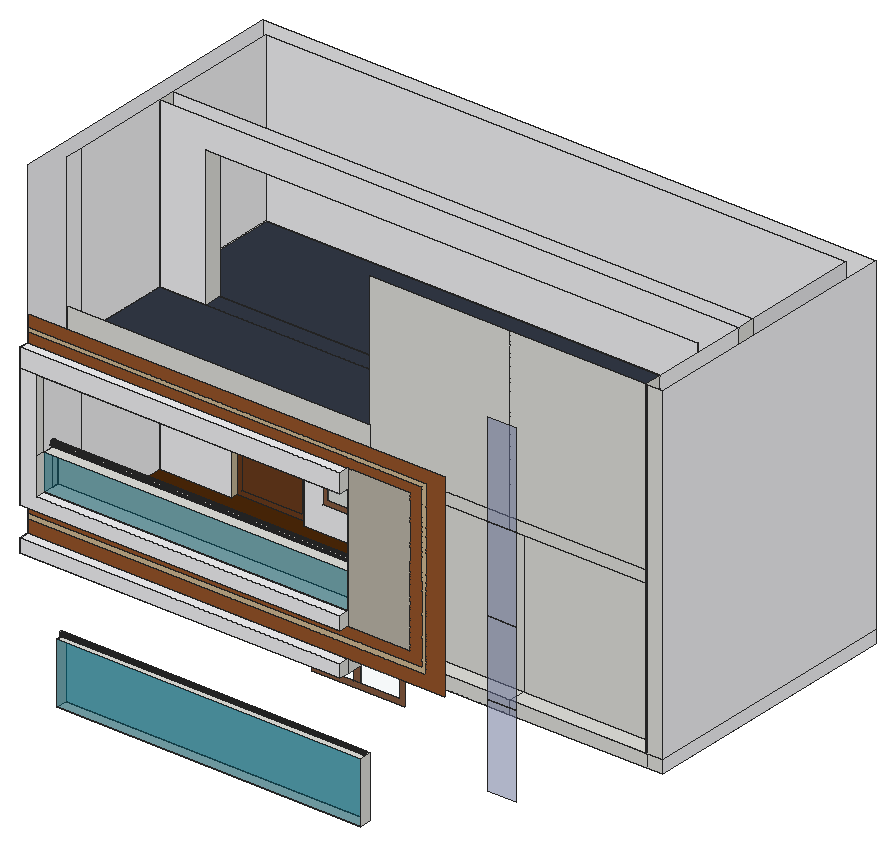
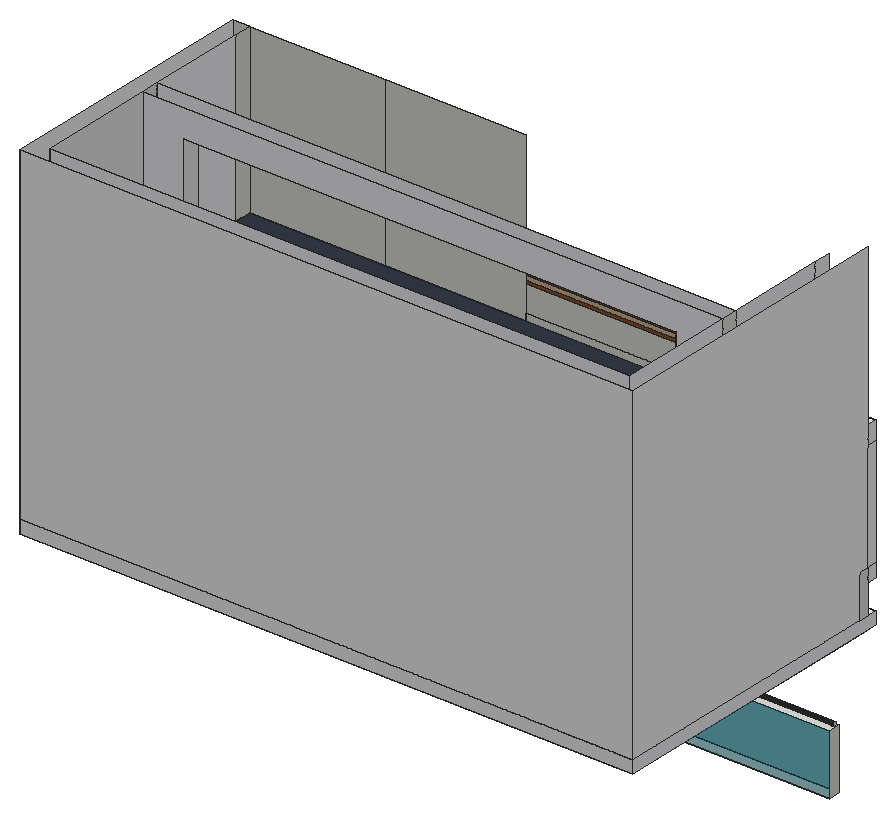
# SketchUp Ruby script. Lengths in inches.
U = 1.inch
M = Sketchup.active_model
def pt(a) = Geom::Point3d.new(a.map { |v| v * U })
def face(e, loops, mat)
  f = e.add_face(loops[0].map { |a| pt(a) })
  loops[1..].each { |l| e.add_face(l.map { |a| pt(a) }).erase! }
  f.material = f.back_material = mat if mat
  f
end
# faces: each face lists its corners as indices into pts; further lists are holes
def faces(e, pts, list, mat = nil) = list.each { |f| face(e, (f[0].is_a?(Array) ? f : [f]).map { |l| l.map { |i| pts[i] } }, mat) }
# xy, xz, yz: faces in a plane at the given z, y or x. An outline is a flat list of corners, or four numbers for a rectangle; further outlines are holes
def ring(l) = l.size == 4 ? [[l[0], l[1]], [l[2], l[1]], [l[2], l[3]], [l[0], l[3]]] : l.each_slice(2).to_a
def flat(e, list, mat, &to3) = list.each { |f| face(e, (f[0].is_a?(Array) ? f : [f]).map { |l| ring(l).map { |u, v| to3.(u, v) } }, mat) }
def xy(e, z, list, mat = nil) = flat(e, list, mat) { |x, y| [x, y, z] }
def xz(e, y, list, mat = nil) = flat(e, list, mat) { |x, z| [x, y, z] }
def yz(e, x, list, mat = nil) = flat(e, list, mat) { |y, z| [x, y, z] }
def lines(e, pts, list) = list.each { |a, b| e.add_line(pt(pts[a]), pt(pts[b])) }
# prism: a flat outline (further loops are holes) pulled along v
def prism(e, loops, v, mat = nil)
  f = face(e, loops, mat); d = Geom::Vector3d.new(v.map { |x| x * U })
  f.pushpull(f.normal.samedirection?(d) ? d.length : -d.length)
end
def box(e, o, s, mat = nil) = prism(e, [[o, [o[0] + s[0], o[1], o[2]], [o[0] + s[0], o[1] + s[1], o[2]], [o[0], o[1] + s[1], o[2]]]], [0, 0, s[2]], mat)
def at(x, y, z, deg = 0) = Geom::Transformation.translation(pt([x, y, z])) * Geom::Transformation.rotation(ORIGIN, Z_AXIS, deg.degrees)
def axes(o, x, y, z) = Geom::Transformation.new([*x, 0, *y, 0, *z, 0, *pt(o).to_a, 1])
def part(name) = M.definitions.add(name)
# library, detail: a bought-in or finely detailed component or shape, given as its bounding box
def library(name, o, s) = part(name).tap { |d| box(d.entities, o, s) }
def detail(e, o, s) = box(e.add_group.entities, o, s)
def put(e, d, t, mat = nil) = e.add_instance(d, t).tap { |i| i.material = mat if mat }
def group(e, t, mat = nil) = e.add_group.tap { |g| g.transformation = t; g.material = mat if mat }.entities
root = M.entities
M.materials.add("[Blinds Vertical Pattern]").color = [245, 245, 247]
M.materials.add("[Blinds Vertical Pattern]2").color = [234, 234, 237]
M.materials.add("[Blinds Vertical Pattern]3").color = [247, 247, 249]
M.materials.add("[Blinds Vertical Pattern]4").color = [245, 245, 247]
M.materials.add("[Cinder Block]1").color = [191, 184, 171]
M.materials.add("[Formica Beige]").color = [211, 187, 149]
M.materials.add("[Leather Red Brown]").color = [76, 40, 8]
M.materials.add("[Quartz Light Brown]").color = [199, 184, 152]
M.materials.add("[Suede Blue]").color = [50, 57, 70]
M.materials.add("[Terrazzo Tile Light]").color = [219, 217, 210]
M.materials.add("[Translucent Glass Safety]").color = [213, 245, 255]
M.materials["[Translucent Glass Safety]"].alpha = 0.12
M.materials.add("[Translucent Glass Sky Reflection]").color = [126, 138, 183]
M.materials["[Translucent Glass Sky Reflection]"].alpha = 0.52
M.materials.add("[Translucent Glass Tinted]").color = [4, 114, 137]
M.materials["[Translucent Glass Tinted]"].alpha = 0.48
M.materials.add("[Wood Cherry Original]").color = [107, 60, 29]
M.materials.add("[Wood Cherry Original]1").color = [152, 86, 42]
M.materials.add("[Wood Veneer 02]").color = [137, 92, 65]
xy(root,284.1875,[[55.41,466.16,415.32,480.02]])
xy(root,356.25,[[55.41,466.16,415.32,480.02]])
xy(root,425.375,[[145.91,609.03,227.47,614.22]],"[Quartz Light Brown]")
xy(root,455.125,[[55.41,446.5625,60.47,455.72],[36.42,455.72,55.41,480.02],[36.42,480.02,55.41,609.03],[742.75,480.02,761.74,609.03],[36.42,609.03,55.41,627.89],
  [55.41,609.03,742.75,627.89],[742.75,609.03,761.74,627.89],[36.42,627.89,55.41,794.75],[55.41,627.89,742.75,775.76],[742.75,627.89,761.74,775.76],
  [55.41,775.76,761.74,794.75]])
xy(root,455.125,[[[36.42,435.375,36.42,455.72,55.41,455.72,55.41,446.5625,60.47,446.5625,60.47,455.72,55.41,455.72,55.41,609.03,742.75,609.03,742.75,480.02,415.32,480.02,415.32,435.375],[62.04,446.5625,67.1,455.72],[68.6,446.5625,73.66,455.72],[88.47,446.5625,93.54,455.72],[102.35,446.5625,107.41,455.72],[95.47,446.5625,100.54,455.72],[75.22,446.5625,80.29,455.72],[109.1,446.5625,114.16,455.72],[81.79,446.5625,86.85,455.72]]],"[Blinds Vertical Pattern]")
xy(root,470.5625,[[36.42,446.5625,36.42,458.64,56.39,458.64,56.39,480.02,415.32,480.02,415.32,446.5625],[36.42,458.64,36.42,794.75,761.74,794.75,761.74,480.02,741.77,480.02,741.77,774.78,56.39,774.78,56.39,458.64],[56.39,480.02,415.32,499.99],[415.32,480.02,580.71,499.99],[580.71,480.02,741.77,499.99],
  [56.39,617.07,56.39,637.38,741.77,637.38,741.77,617.07,226.6875,617.07,226.6875,624.63,141.37,624.63,141.37,617.07],[56.39,637.38,741.77,774.78]])
xy(root,470.5625,[[36.42,435.375,415.32,446.5625]],"[Blinds Vertical Pattern]")
xy(root,470.5625,[[56.39,499.99,741.77,499.99,741.77,617.07,226.6875,617.07,226.6875,624.63,141.37,624.63,141.37,617.07,56.39,617.07]],"[Leather Red Brown]")
xy(root,505.3125,[[36.42,435.375,415.32,446.5625]])
xy(root,521.375,[[56.39,446.5625,415.32,467.14]])
xy(root,521.375,[[56.39,435.375,415.32,446.5625]],"[Blinds Vertical Pattern]")
xy(root,521.375,[[56.39,467.14,415.32,480.02]],"[Translucent Glass Tinted]")
xy(root,564.1875,[[56.39,446.5625,415.32,467.14]])
xy(root,612.8125,[[141.37,617.07,226.6875,624.63]],"[Quartz Light Brown]")
xy(root,650.5625,[[36.42,435.375,56.39,446.5625],[415.32,480.02,580.71,499.99],[580.71,480.02,741.77,499.99],[56.39,617.07,741.77,637.38],[56.39,637.38,741.77,774.78]])
xy(root,650.5625,[[56.39,435.375,56.39,617.07,741.77,617.07,741.77,499.99,415.32,499.99,415.32,435.375]],"[Blinds Vertical Pattern]")
xy(root,664.4375,[[56.39,617.07,111.4,637.38],[693.46,617.07,741.77,637.38]])
xy(root,664.4375,[[56.39,480.02,741.77,617.07],[111.4,617.07,693.46,637.38],[56.39,637.38,741.77,774.78]],"[Suede Blue]")
xy(root,672.8125,[[56.39,446.5625,415.32,480.02]])
xy(root,672.8125,[[36.42,435.375,415.32,446.5625]],"[Blinds Vertical Pattern]")
xz(root,435.375,[[36.42,455.125,415.32,470.5625],[36.42,505.3125,415.32,505.3125,415.32,521.375,56.39,521.375,56.39,650.5625,36.42,650.5625],[36.42,650.5625,415.32,672.8125]],"[Blinds Vertical Pattern]")
xz(root,446.5625,[[36.42,505.3125,36.42,650.5625,56.39,650.5625,56.39,521.375,415.32,521.375,415.32,505.3125],[36.42,650.5625,56.39,672.8125]])
xz(root,446.5625,[[415.32,505.3125,489.38,672.8125]],"[Cinder Block]1")
xz(root,446.5625,[[36.42,486.3125,507.82,486.3125,507.82,689.0625,36.42,689.0625,36.42,683.75,503.58,683.75,503.58,492.6875,36.42,492.6875]],"[Formica Beige]")
xz(root,446.5625,[[580.71,387.88,615.19,485.6],[580.71,485.6,615.19,574.11],[580.71,574.11,615.19,674.03],[580.71,674.03,615.19,785.52]],"[Translucent Glass Sky Reflection]")
xz(root,446.5625,[[56.39,521.375,415.32,564.1875]],"[Translucent Glass Tinted]")
xz(root,446.5625,[[36.42,470.5625,530.38,470.5625,530.38,703.5,36.42,703.5,36.42,689.0625,507.82,689.0625,507.82,486.3125,36.42,486.3125],[36.42,492.6875,503.58,492.6875,503.58,683.75,36.42,683.75,36.42,672.8125,489.38,672.8125,489.38,505.3125,36.42,505.3125]],"[Wood Cherry Original]1")
xz(root,458.64,[[36.42,470.5625,56.39,505.3125],[36.42,505.3125,56.39,521.375]])
xz(root,466.16,[[55.41,284.1875,415.32,356.25]],"[Translucent Glass Tinted]")
xz(root,467.14,[[56.39,521.375,415.32,564.1875]])
xz(root,480.02,[[415.32,455.125,580.71,470.5625],[580.71,455.125,742.75,470.5625],[742.75,455.125,761.74,470.5625],[56.39,470.5625,415.32,505.3125],[741.77,470.5625,742.75,861.625],
  [742.75,470.5625,761.74,861.625],[56.39,505.3125,415.32,521.375],[415.32,650.5625,580.71,664.4375],[580.71,650.5625,741.77,664.4375],[56.39,664.4375,415.32,672.8125],
  [415.32,664.4375,580.71,861.625],[580.71,664.4375,741.77,861.625],[56.39,672.8125,415.32,703.5]])
xz(root,480.02,[[55.41,284.1875,415.32,356.25]],"[Translucent Glass Tinted]")
xz(root,499.99,[[415.32,470.5625,580.71,650.5625],[580.71,470.5625,741.77,650.5625]])
xz(root,609.03,[[250.07,332.88,293.02,420.74],[301.15,332.88,346.58,420.74]],"[Translucent Glass Safety]")
xz(root,609.03,[[[243.47,326.28,353.18,427.34],[250.07,332.88,346.58,420.74]],[293.02,332.88,301.15,420.74]],"[Wood Veneer 02]")
xz(root,617.07,[[56.39,650.5625,741.77,664.4375]])
xz(root,617.07,[[[56.39,470.5625,141.37,470.5625,141.37,612.8125,226.6875,612.8125,226.6875,470.5625,741.77,470.5625,741.77,650.5625,56.39,650.5625],[249.8,500.52,354.17,613.9]],[56.39,664.4375,111.4,664.4375,111.4,828.25,693.46,828.25,693.46,664.4375,741.77,664.4375,741.77,861.625,56.39,861.625]],"[Blinds Vertical Pattern]")
xz(root,617.07,[[256.05,506.78,298.04,607.64],[307.09,506.78,347.92,607.64]],"[Translucent Glass Safety]")
xz(root,617.07,[[[249.8,500.52,354.17,613.9],[256.05,506.78,347.92,607.64]],[298.04,506.78,307.09,607.64]],"[Wood Veneer 02]")
xz(root,624.63,[[[141.37,470.5625,226.6875,612.8125],[147.76,476.95,220.3,606.43]],[147.76,476.95,220.3,606.43]],"[Wood Cherry Original]")
xz(root,637.38,[[56.39,470.5625,741.77,650.5625],[56.39,650.5625,741.77,664.4375]])
xz(root,637.38,[[56.39,664.4375,56.39,861.625,741.77,861.625,741.77,664.4375,693.46,664.4375,693.46,828.25,111.4,828.25,111.4,664.4375]],"[Blinds Vertical Pattern]4")
xz(root,774.78,[[56.39,470.5625,741.77,650.5625],[56.39,650.5625,741.77,664.4375]])
xz(root,774.78,[[56.39,664.4375,741.77,861.625]],"[Blinds Vertical Pattern]")
xz(root,794.75,[[36.42,455.125,761.74,470.5625],[36.42,470.5625,761.74,861.625]],"[Blinds Vertical Pattern]3")
yz(root,36.42,[[446.5625,470.5625,458.64,521.375]])
yz(root,36.42,[[435.375,455.125,794.75,470.5625],[435.375,505.3125,446.5625,521.375],[435.375,521.375,446.5625,650.5625],[435.375,650.5625,446.5625,672.8125]],"[Blinds Vertical Pattern]")
yz(root,36.42,[[458.64,470.5625,458.64,521.375,446.5625,521.375,446.5625,861.625,794.75,861.625,794.75,470.5625]],"[Blinds Vertical Pattern]3")
yz(root,55.41,[[466.16,284.1875,480.02,356.25],[472.17,357.99,471.66,358.05,471.17,358.25,470.76,358.57,470.44,358.99,470.24,359.47,470.17,359.99,470.24,360.5,470.44,360.99,470.76,361.4,471.17,361.72,471.66,361.92,472.17,361.99,472.69,361.92,473.17,361.72,473.59,361.4,473.91,360.99,474.11,360.5,474.17,359.99,474.11,359.47,473.91,358.99,473.59,358.57,473.17,358.25,472.69,358.05]])
yz(root,56.39,[[458.64,470.5625,480.02,505.3125],[617.07,470.5625,637.38,650.5625],[637.38,470.5625,774.78,650.5625],[458.64,505.3125,480.02,521.375],[435.375,521.375,446.5625,564.1875],
  [446.5625,521.375,458.64,564.1875],[458.64,521.375,467.14,564.1875],[435.375,564.1875,446.5625,650.5625],[457.67,566.14,456.85,566.25,456.08,566.57,455.42,567.07,454.91,567.73,454.59,568.5,454.49,569.33,454.59,570.15,454.91,570.92,455.42,571.58,456.08,572.09,456.85,572.41,457.67,572.51,458.5,572.41,459.27,572.09,459.93,571.58,460.43,570.92,460.75,570.15,460.86,569.33,460.75,568.5,460.43,567.73,459.93,567.07,459.27,566.57,458.5,566.25],[446.5625,650.5625,480.02,672.8125],
  [480.02,650.5625,499.99,664.4375],[499.99,650.5625,617.07,664.4375],[617.07,650.5625,637.38,664.4375],[637.38,650.5625,774.78,664.4375],[617.07,664.4375,637.38,861.625]])
yz(root,56.39,[[[480.02,470.5625,499.99,470.5625,499.99,650.5625,446.5625,650.5625,446.5625,564.1875,467.14,564.1875,467.14,521.375,480.02,521.375],[457.67,566.14,456.85,566.25,456.08,566.57,455.42,567.07,454.91,567.73,454.59,568.5,454.49,569.33,454.59,570.15,454.91,570.92,455.42,571.58,456.08,572.09,456.85,572.41,457.67,572.51,458.5,572.41,459.27,572.09,459.93,571.58,460.43,570.92,460.75,570.15,460.86,569.33,460.75,568.5,460.43,567.73,459.93,567.07,459.27,566.57,458.5,566.25]],[499.99,470.5625,617.07,650.5625],[480.02,664.4375,499.99,861.625],[499.99,664.4375,617.07,861.625],[637.38,664.4375,774.78,861.625]],"[Blinds Vertical Pattern]")
yz(root,111.4,[[617.07,664.4375,637.38,828.25]])
yz(root,141.37,[[617.07,470.5625,624.63,612.8125]],"[Quartz Light Brown]")
yz(root,226.6875,[[617.07,470.5625,624.63,612.8125]],"[Quartz Light Brown]")
yz(root,415.32,[[466.16,284.1875,480.02,356.25],[435.375,455.125,446.5625,470.5625],[446.5625,455.125,480.02,470.5625],[435.375,505.3125,446.5625,521.375],[446.5625,505.3125,480.02,521.375],
  [446.5625,521.375,467.14,564.1875],[435.375,650.5625,446.5625,672.8125],[446.5625,650.5625,480.02,672.8125]])
yz(root,415.32,[[[480.02,470.5625,480.02,521.375,467.14,521.375,467.14,564.1875,446.5625,564.1875,446.5625,650.5625,499.99,650.5625,499.99,470.5625],[457.67,566.14,458.5,566.25,459.27,566.57,459.93,567.07,460.43,567.73,460.75,568.5,460.86,569.33,460.75,570.15,460.43,570.92,459.93,571.58,459.27,572.09,458.5,572.41,457.67,572.51,456.85,572.41,456.08,572.09,455.42,571.58,454.91,570.92,454.59,570.15,454.49,569.33,454.59,568.5,454.91,567.73,455.42,567.07,456.08,566.57,456.85,566.25]]],"[Blinds Vertical Pattern]2")
yz(root,693.46,[[617.07,664.4375,637.38,828.25]],"[Blinds Vertical Pattern]2")
yz(root,741.77,[[480.02,470.5625,499.99,650.5625],[617.07,470.5625,637.38,650.5625],[637.38,470.5625,774.78,650.5625],[480.02,650.5625,499.99,664.4375],[499.99,650.5625,617.07,664.4375],
  [617.07,650.5625,637.38,664.4375],[637.38,650.5625,774.78,664.4375],[480.02,664.4375,499.99,861.625],[617.07,664.4375,637.38,861.625]])
yz(root,741.77,[[499.99,470.5625,617.07,650.5625],[499.99,664.4375,617.07,861.625]],"[Blinds Vertical Pattern]")
yz(root,741.77,[[637.38,664.4375,774.78,861.625]],"[Blinds Vertical Pattern]2")
yz(root,761.74,[[480.02,455.125,794.75,470.5625],[480.02,470.5625,794.75,861.625]],"[Blinds Vertical Pattern]3")
p = [[55.41,471.66,358.05],[55.41,472.17,357.99],[415.32,472.17,357.99],[415.32,471.66,358.05],[55.41,472.69,358.05],[415.32,472.69,358.05],
  [55.41,471.17,358.25],[415.32,471.17,358.25],[55.41,473.17,358.25],[415.32,473.17,358.25],[55.41,470.76,358.57],[415.32,470.76,358.57],
  [55.41,473.59,358.57],[415.32,473.59,358.57],[55.41,470.44,358.99],[415.32,470.44,358.99],[55.41,473.91,358.99],[415.32,473.91,358.99],
  [55.41,470.24,359.47],[415.32,470.24,359.47],[55.41,474.11,359.47],[415.32,474.11,359.47],[55.41,470.17,359.99],[415.32,470.17,359.99],
  [55.41,474.17,359.99],[415.32,474.17,359.99],[55.41,470.24,360.5],[415.32,470.24,360.5],[55.41,474.11,360.5],[415.32,474.11,360.5],
  [55.41,470.44,360.99],[415.32,470.44,360.99],[55.41,473.91,360.99],[415.32,473.91,360.99],[55.41,470.76,361.4],[415.32,470.76,361.4],
  [55.41,473.59,361.4],[415.32,473.59,361.4],[55.41,471.17,361.72],[415.32,471.17,361.72],[55.41,473.17,361.72],[415.32,473.17,361.72],
  [55.41,471.66,361.92],[415.32,471.66,361.92],[55.41,472.69,361.92],[415.32,472.69,361.92],[55.41,472.17,361.99],[415.32,472.17,361.99],
  [56.39,456.85,566.25],[56.39,457.67,566.14],[415.32,457.67,566.14],[415.32,456.85,566.25],[56.39,458.5,566.25],[415.32,458.5,566.25],
  [56.39,456.08,566.57],[415.32,456.08,566.57],[56.39,459.27,566.57],[415.32,459.27,566.57],[56.39,455.42,567.07],[415.32,455.42,567.07],
  [56.39,459.93,567.07],[415.32,459.93,567.07],[56.39,454.91,567.73],[415.32,454.91,567.73],[56.39,460.43,567.73],[415.32,460.43,567.73],
  [56.39,454.59,568.5],[415.32,454.59,568.5],[56.39,460.75,568.5],[415.32,460.75,568.5],[56.39,454.49,569.33],[415.32,454.49,569.33],
  [56.39,460.86,569.33],[415.32,460.86,569.33],[56.39,454.59,570.15],[415.32,454.59,570.15],[56.39,460.75,570.15],[415.32,460.75,570.15],
  [56.39,454.91,570.92],[415.32,454.91,570.92],[56.39,460.43,570.92],[415.32,460.43,570.92],[56.39,455.42,571.58],[415.32,455.42,571.58],
  [56.39,459.93,571.58],[415.32,459.93,571.58],[56.39,456.08,572.09],[415.32,456.08,572.09],[56.39,459.27,572.09],[415.32,459.27,572.09],
  [56.39,456.85,572.41],[415.32,456.85,572.41],[56.39,458.5,572.41],[415.32,458.5,572.41],[56.39,457.67,572.51],[415.32,457.67,572.51]]
faces(root,p,[[0,1,2,3],[1,4,5,2],[6,0,3,7],[4,8,9,5],[10,6,7,11],[8,12,13,9],[14,10,11,15],[12,16,17,13],
  [18,14,15,19],[16,20,21,17],[22,18,19,23],[20,24,25,21],[26,22,23,27],[24,28,29,25],[30,26,27,31],[28,32,33,29],
  [34,30,31,35],[32,36,37,33],[38,34,35,39],[36,40,41,37],[42,38,39,43],[40,44,45,41],[46,42,43,47],[44,46,47,45],
  [48,49,50,51],[49,52,53,50],[54,48,51,55],[52,56,57,53],[58,54,55,59],[56,60,61,57],[62,58,59,63],[60,64,65,61],
  [66,62,63,67],[64,68,69,65],[70,66,67,71],[68,72,73,69],[74,70,71,75],[72,76,77,73],[78,74,75,79],[76,80,81,77],
  [82,78,79,83],[80,84,85,81],[86,82,83,87],[84,88,89,85],[90,86,87,91],[88,92,93,89],[94,90,91,95],[92,94,95,93]],"[Terrazzo Tile Light]")
